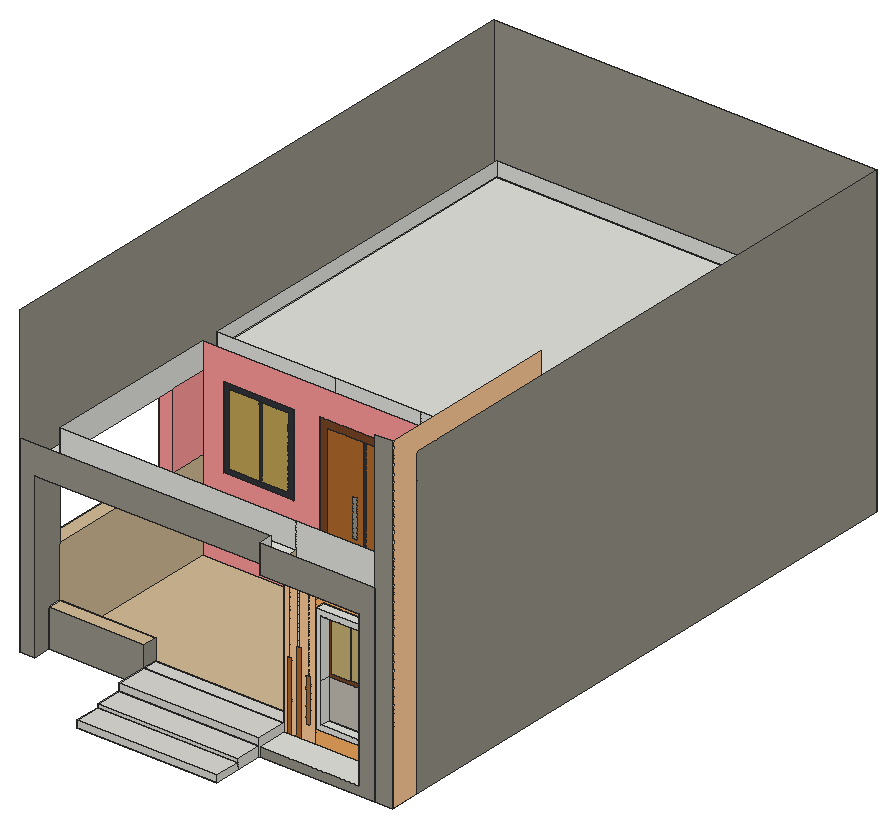
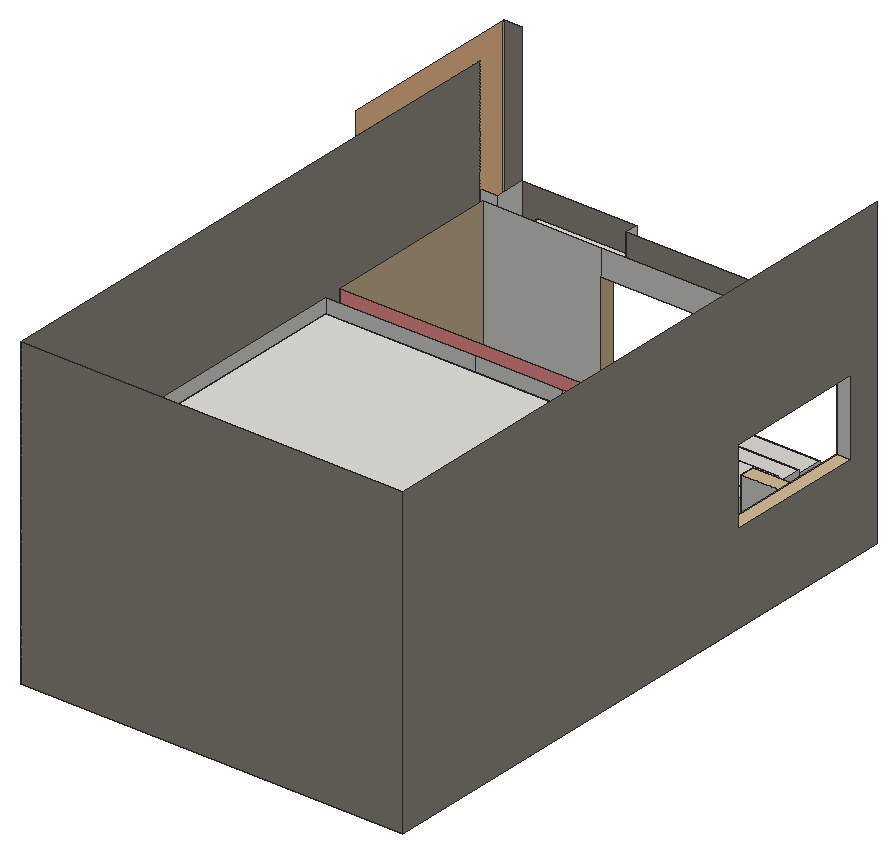
# SketchUp Ruby script. Lengths in inches.
U = 1.inch
M = Sketchup.active_model
def pt(a) = Geom::Point3d.new(a.map { |v| v * U })
def face(e, loops, mat)
  f = e.add_face(loops[0].map { |a| pt(a) })
  loops[1..].each { |l| e.add_face(l.map { |a| pt(a) }).erase! }
  f.material = f.back_material = mat if mat
  f
end
# faces: each face lists its corners as indices into pts; further lists are holes
def faces(e, pts, list, mat = nil) = list.each { |f| face(e, (f[0].is_a?(Array) ? f : [f]).map { |l| l.map { |i| pts[i] } }, mat) }
# xy, xz, yz: faces in a plane at the given z, y or x. An outline is a flat list of corners, or four numbers for a rectangle; further outlines are holes
def ring(l) = l.size == 4 ? [[l[0], l[1]], [l[2], l[1]], [l[2], l[3]], [l[0], l[3]]] : l.each_slice(2).to_a
def flat(e, list, mat, &to3) = list.each { |f| face(e, (f[0].is_a?(Array) ? f : [f]).map { |l| ring(l).map { |u, v| to3.(u, v) } }, mat) }
def xy(e, z, list, mat = nil) = flat(e, list, mat) { |x, y| [x, y, z] }
def xz(e, y, list, mat = nil) = flat(e, list, mat) { |x, z| [x, y, z] }
def yz(e, x, list, mat = nil) = flat(e, list, mat) { |y, z| [x, y, z] }
def lines(e, pts, list) = list.each { |a, b| e.add_line(pt(pts[a]), pt(pts[b])) }
# prism: a flat outline (further loops are holes) pulled along v
def prism(e, loops, v, mat = nil)
  f = face(e, loops, mat); d = Geom::Vector3d.new(v.map { |x| x * U })
  f.pushpull(f.normal.samedirection?(d) ? d.length : -d.length)
end
def box(e, o, s, mat = nil) = prism(e, [[o, [o[0] + s[0], o[1], o[2]], [o[0] + s[0], o[1] + s[1], o[2]], [o[0], o[1] + s[1], o[2]]]], [0, 0, s[2]], mat)
def at(x, y, z, deg = 0) = Geom::Transformation.translation(pt([x, y, z])) * Geom::Transformation.rotation(ORIGIN, Z_AXIS, deg.degrees)
def axes(o, x, y, z) = Geom::Transformation.new([*x, 0, *y, 0, *z, 0, *pt(o).to_a, 1])
def part(name) = M.definitions.add(name)
# library, detail: a bought-in or finely detailed component or shape, given as its bounding box
def library(name, o, s) = part(name).tap { |d| box(d.entities, o, s) }
def detail(e, o, s) = box(e.add_group.entities, o, s)
def put(e, d, t, mat = nil) = e.add_instance(d, t).tap { |i| i.material = mat if mat }
def group(e, t, mat = nil) = e.add_group.tap { |g| g.transformation = t; g.material = mat if mat }.entities
root = M.entities
M.materials.add("[Blinds Cloth Horizontal]").color = [192, 163, 85]
M.materials.add("[Color A02]").color = [255, 153, 153]
M.materials.add("[Color C02]").color = [255, 204, 153]
M.materials.add("[Color C03]").color = [255, 178, 101]
M.materials.add("[Field Rectangle Tile]").color = [196, 189, 179]
M.materials.add("[Formica Beige]").color = [211, 187, 149]
M.materials.add("[Formica Graystone]").color = [149, 146, 135]
M.materials.add("[Formica Laminate Dark]").color = [50, 53, 60]
M.materials.add("[Terrazzo Tile Light]").color = [219, 217, 210]
M.materials.add("[Window Covering 02]").color = [199, 178, 115]
M.materials.add("[Wood Bamboo]").color = [177, 105, 43]
M.materials.add("[Wood Veneer 01]").color = [120, 70, 37]
xy(root,0,[[68.8,0,156.76,16.17],[68.8,16.17,156.76,32.77],[68.8,32.77,156.76,52.39],[156.76,33.14,228.875,52.39],[228.875,33.14,240,52.39],
  [0,41.58,9,61.39],[9,52.39,68.8,61.39],[68.8,52.39,156.76,61.39],[156.76,52.39,156.76,61.39,231,61.39,231,172.96,240,172.96,240,52.39],[0,61.39,9,172.96],
  [0,172.96,82.72,184.44],[82.72,172.96,137.09,184.44],[137.09,172.96,240,184.44],[0,184.44,0,412.39,240,412.39,240,184.44,231,184.44,231,403.39,9,403.39,9,184.44],[9,184.44,231,403.39]])
xy(root,0,[[9,61.39,231,172.96]],"[Formica Beige]")
xy(root,4.0625,[[68.8,0,156.76,16.17]],"[Terrazzo Tile Light]")
xy(root,5.53,[[156.76,33.14,218.92,52.39]])
xy(root,6,[[68.8,16.17,156.76,32.77]],"[Terrazzo Tile Light]")
xy(root,10.375,[[68.8,32.77,156.76,52.39],[68.8,52.39,156.76,61.39]],"[Terrazzo Tile Light]")
xy(root,18.38,[[181.34,46.45,214.03,52.39]])
xy(root,21.61,[[184.57,46.45,210.8,52.39]])
xy(root,23.5,[[9,52.39,68.8,61.39]],"[Formica Beige]")
xy(root,50.59,[[22.41,172.96,66.1,184.44]])
xy(root,55.875,[[0,61.39,9,149.96]],"[Formica Beige]")
xy(root,83.1,[[184.57,46.45,210.8,52.39]])
xy(root,86.32,[[181.34,46.45,214.03,52.39]])
xy(root,102.15,[[156.76,33.14,218.92,52.39],[9,41.58,156.76,52.39],[22.41,172.96,66.1,184.44]])
xy(root,103.1875,[[82.72,172.96,137.09,184.44]])
xy(root,103.45,[[0,61.39,9,149.96]])
xy(root,111,[[9,184.44,231,403.39]])
xz(root,0,[[68.8,0,156.76,4.0625]],"[Terrazzo Tile Light]")
xz(root,16.17,[[68.8,0,156.76,4.0625]])
xz(root,16.17,[[68.8,4.0625,156.76,6]],"[Terrazzo Tile Light]")
xz(root,32.77,[[68.8,0,156.76,6]])
xz(root,32.77,[[68.8,6,156.76,10.375]],"[Terrazzo Tile Light]")
xz(root,33.14,[[156.76,0,228.875,0,228.875,120,156.76,120,156.76,102.15,218.92,102.15,218.92,5.53,156.76,5.53],[228.875,0,240,206.25]],"[Formica Graystone]")
xz(root,41.58,[[0,0,9,0,9,102.15,156.76,102.15,156.76,120,0,120]],"[Formica Graystone]")
xz(root,46.45,[[[181.34,18.38,214.03,86.32],[184.57,21.61,210.8,83.1]]])
xz(root,52.39,[[68.8,0,156.76,10.375],[228.875,0,240,120],[[181.34,18.38,214.03,86.32],[184.57,21.61,210.8,83.1]],[171.93,42.41,172.42,102.15],[159.7,48.66,160.48,102.15],
  [165.48,56.61,166.06,102.15]])
xz(root,52.39,[[156.76,5.53,158.13,5.53,158.13,48.66,159.7,48.66,159.7,102.15,156.76,102.15],[161.26,5.53,164.3125,5.53,164.3125,56.61,165.48,56.61,165.48,102.15,160.48,102.15,160.48,48.66,161.26,48.66],[167.71,5.53,176.52,5.53,176.52,102.15,172.42,102.15,172.42,42.41,173.64,42.41,173.64,14.52,170.21,14.52,170.21,42.41,171.93,42.41,171.93,102.15,166.06,102.15,166.06,56.61,167.71,56.61]],"[Color C02]")
xz(root,52.39,[[[176.52,5.53,218.92,102.15],[181.34,18.38,214.03,86.32]]],"[Color C03]")
xz(root,52.39,[[184.57,21.61,210.8,46.24]],"[Field Rectangle Tile]")
xz(root,52.39,[[9,0,68.8,23.5]],"[Formica Graystone]")
xz(root,52.39,[[186.94,48.61,197.68,80.72],[199.01,48.61,208.43,80.72]],"[Window Covering 02]")
xz(root,52.39,[[158.13,5.53,161.26,48.66],[164.3125,5.53,167.71,56.61],[170.21,14.52,173.64,42.41]],"[Wood Bamboo]")
xz(root,52.39,[[[184.57,46.24,210.8,83.1],[186.94,48.61,208.43,80.72]],[197.68,48.61,199.01,80.72]],"[Wood Veneer 01]")
xz(root,61.39,[[9,0,68.8,23.5],[68.8,0,156.76,10.375],[156.76,0,231,120],[0,55.875,9,103.45],[9,103.45,156.76,120]])
xz(root,149.96,[[0,55.875,9,103.45]],"[Color A02]")
xz(root,172.96,[[25.9375,54.11,44.26,98.63],[46.52,54.11,62.58,98.63]],"[Blinds Cloth Horizontal]")
xz(root,172.96,[[[9,0,82.72,0,82.72,103.1875,137.09,103.1875,137.09,0,231,0,231,120,9,120],[22.41,50.59,66.1,102.15]]],"[Color A02]")
xz(root,172.96,[[103.04,42.65,106.1,65.84],[117.35,42.65,120.41,65.84]],"[Formica Graystone]")
xz(root,172.96,[[109.9,4.24,111.36,98.95],[[22.41,50.59,66.1,102.15],[25.9375,54.11,62.58,98.63]],[44.26,54.11,46.52,98.63]],"[Formica Laminate Dark]")
xz(root,172.96,[[[86.96,4.24,109.9,98.95],[103.04,42.65,106.1,65.84]],[[111.36,4.24,132.85,98.95],[117.35,42.65,120.41,65.84]]],"[Wood Bamboo]")
xz(root,172.96,[[[82.72,0,137.09,103.1875],[86.96,4.24,132.85,98.95]]],"[Wood Veneer 01]")
xz(root,184.44,[[[9,0,9,111,231,111,231,0,137.09,0,137.09,103.1875,82.72,103.1875,82.72,0],[22.41,50.59,66.1,102.15]],[9,111,82.72,120],[82.72,111,137.09,120],[137.09,111,231,120]])
xz(root,403.39,[[9,0,231,111],[9,111,231,120]])
xz(root,412.39,[[0,0,240,192]],"[Formica Graystone]")
yz(root,0,[[[41.58,0,412.39,192],[61.39,55.875,149.96,103.45]]],"[Formica Graystone]")
yz(root,9,[[52.39,0,61.39,23.5],[184.44,0,403.39,111],[61.39,103.45,172.96,120],[184.44,111,403.39,120]])
yz(root,9,[[149.96,55.875,172.96,103.45]],"[Color A02]")
yz(root,9,[[61.39,0,172.96,55.875]],"[Formica Beige]")
yz(root,9,[[41.58,0,52.39,0,52.39,23.5,61.39,23.5,61.39,103.45,52.39,102.15,41.58,102.15]],"[Formica Graystone]")
yz(root,22.41,[[172.96,50.59,184.44,102.15]])
yz(root,66.1,[[172.96,50.59,184.44,102.15]])
yz(root,68.8,[[52.39,0,61.39,10.375]])
yz(root,68.8,[[52.39,10.375,61.39,23.5]],"[Formica Graystone]")
yz(root,68.8,[[0,0,16.17,4.0625],[16.17,0,32.77,6],[32.77,0,52.39,10.375]],"[Terrazzo Tile Light]")
yz(root,82.72,[[172.96,0,184.44,103.1875]])
yz(root,137.09,[[172.96,0,184.44,103.1875]])
yz(root,156.76,[[52.39,0,61.39,10.375],[33.14,102.15,41.58,120]])
yz(root,156.76,[[52.39,10.375,52.39,102.15,61.39,103.45,61.39,10.375]],"[Formica Beige]")
yz(root,156.76,[[0,0,16.17,4.0625],[16.17,0,32.77,6],[32.77,0,33.14,0,33.14,5.53,52.39,5.53,52.39,10.375,32.77,10.375]],"[Terrazzo Tile Light]")
yz(root,181.34,[[46.45,18.38,52.39,86.32]])
yz(root,184.57,[[46.45,21.61,52.39,46.24],[46.45,46.24,52.39,83.1]])
yz(root,210.8,[[46.45,21.61,52.39,46.24],[46.45,46.24,52.39,83.1]])
yz(root,214.03,[[46.45,18.38,52.39,86.32]])
yz(root,218.92,[[33.14,5.53,52.39,102.15]],"[Formica Beige]")
yz(root,228.875,[[33.14,0,52.39,120]])
yz(root,231,[[184.44,0,403.39,111],[184.44,111,403.39,120]])
yz(root,231,[[61.39,0,172.96,120]],"[Formica Beige]")
yz(root,240,[[33.14,0,34.33,206.25]])
yz(root,240,[[34.33,0,52.39,0,52.39,192,149.14,192,149.14,206.25,34.33,206.25]],"[Color C02]")
yz(root,240,[[52.39,0,412.39,192]],"[Formica Graystone]")
p = [[9,52.39,102.15],[9,61.39,103.45],[156.76,61.39,103.45],[156.76,52.39,102.15]]
faces(root,p,[[0,1,2,3]])
